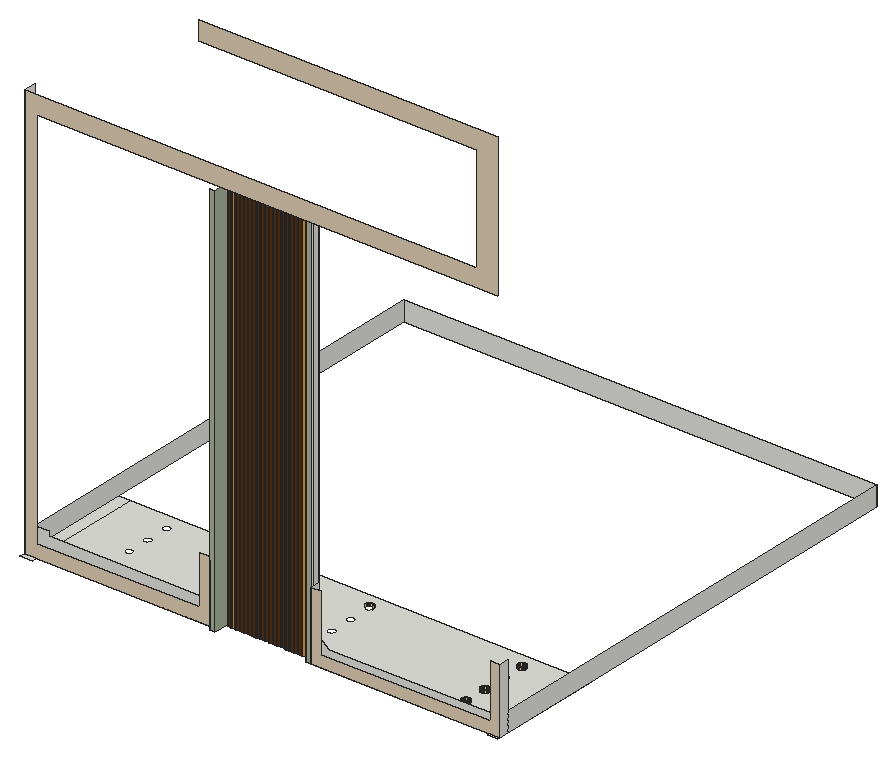
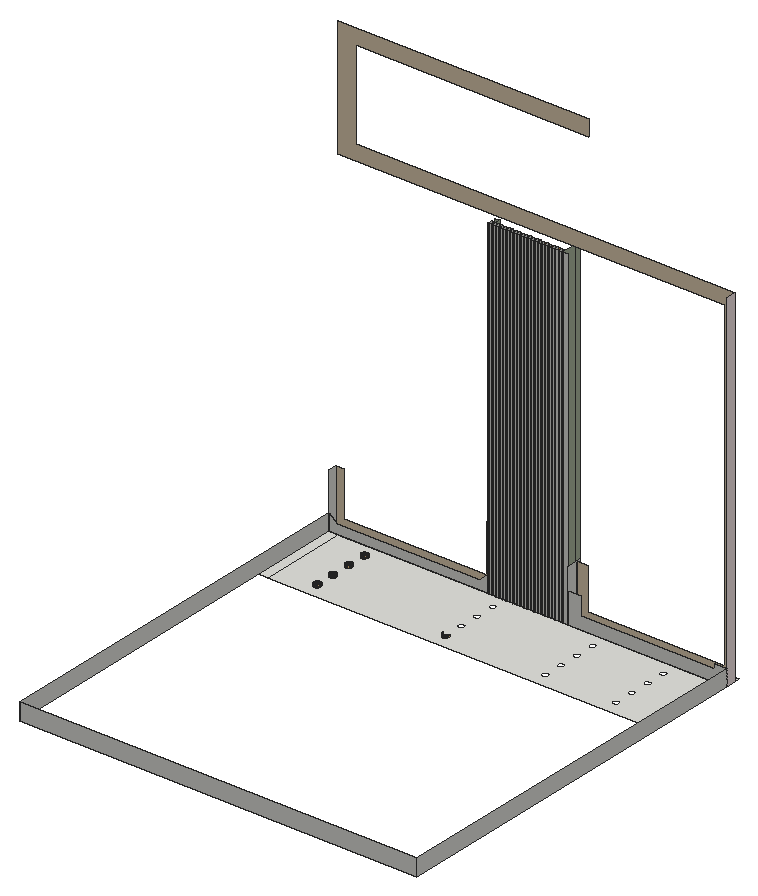
# SketchUp Ruby script. Lengths in inches.
U = 1.inch
M = Sketchup.active_model
def pt(a) = Geom::Point3d.new(a.map { |v| v * U })
def face(e, loops, mat)
  f = e.add_face(loops[0].map { |a| pt(a) })
  loops[1..].each { |l| e.add_face(l.map { |a| pt(a) }).erase! }
  f.material = f.back_material = mat if mat
  f
end
# faces: each face lists its corners as indices into pts; further lists are holes
def faces(e, pts, list, mat = nil) = list.each { |f| face(e, (f[0].is_a?(Array) ? f : [f]).map { |l| l.map { |i| pts[i] } }, mat) }
# xy, xz, yz: faces in a plane at the given z, y or x. An outline is a flat list of corners, or four numbers for a rectangle; further outlines are holes
def ring(l) = l.size == 4 ? [[l[0], l[1]], [l[2], l[1]], [l[2], l[3]], [l[0], l[3]]] : l.each_slice(2).to_a
def flat(e, list, mat, &to3) = list.each { |f| face(e, (f[0].is_a?(Array) ? f : [f]).map { |l| ring(l).map { |u, v| to3.(u, v) } }, mat) }
def xy(e, z, list, mat = nil) = flat(e, list, mat) { |x, y| [x, y, z] }
def xz(e, y, list, mat = nil) = flat(e, list, mat) { |x, z| [x, y, z] }
def yz(e, x, list, mat = nil) = flat(e, list, mat) { |y, z| [x, y, z] }
def lines(e, pts, list) = list.each { |a, b| e.add_line(pt(pts[a]), pt(pts[b])) }
# prism: a flat outline (further loops are holes) pulled along v
def prism(e, loops, v, mat = nil)
  f = face(e, loops, mat); d = Geom::Vector3d.new(v.map { |x| x * U })
  f.pushpull(f.normal.samedirection?(d) ? d.length : -d.length)
end
def box(e, o, s, mat = nil) = prism(e, [[o, [o[0] + s[0], o[1], o[2]], [o[0] + s[0], o[1] + s[1], o[2]], [o[0], o[1] + s[1], o[2]]]], [0, 0, s[2]], mat)
def at(x, y, z, deg = 0) = Geom::Transformation.translation(pt([x, y, z])) * Geom::Transformation.rotation(ORIGIN, Z_AXIS, deg.degrees)
def axes(o, x, y, z) = Geom::Transformation.new([*x, 0, *y, 0, *z, 0, *pt(o).to_a, 1])
def part(name) = M.definitions.add(name)
# library, detail: a bought-in or finely detailed component or shape, given as its bounding box
def library(name, o, s) = part(name).tap { |d| box(d.entities, o, s) }
def detail(e, o, s) = box(e.add_group.entities, o, s)
def put(e, d, t, mat = nil) = e.add_instance(d, t).tap { |i| i.material = mat if mat }
def group(e, t, mat = nil) = e.add_group.tap { |g| g.transformation = t; g.material = mat if mat }.entities
root = M.entities
M.materials.add("Generic").color = [90, 50, 18]
M.materials.add("Generic\#2").color = [245, 199, 133]
M.materials.add("Generic\#4").color = [232, 149, 60]
M.materials.add("Generic\#6").color = [223, 205, 179]
M.materials.add("Generic\#8").color = [168, 180, 155]
M.materials.add("Generic\#9").color = [246, 231, 231]
xy(root,120,[[2.3125,34.9375,15.4375,41],[204.09,35.5625,210.09,54.5625],[2.3125,41,15.4375,54.5625],[15.4375,41,204.09,54.5625],[497,41,507.875,43.625],
  [300.09,43.625,300.09,54.5625,300.47,54.5625,300.47,49.875,304.47,49.875,304.47,54.5625,306.09,54.5625,306.09,43.625],[306.09,43.625,497,54.5625],[497,43.625,507.875,54.5625],[211.72,49.875,215.72,54.5625],[300.47,49.875,304.47,54.5625],
  [2.3125,54.5625,15.4375,166.1875],[[15.4375,54.5625,497,166.1875],[448.19,68.72,449.28,68.86,450.29,69.28,451.15,69.95,451.82,70.8125,452.24,71.82,452.38,72.91,452.24,73.99,451.82,75,451.15,75.87,450.29,76.53,449.28,76.95,448.19,77.09,447.11,76.95,446.1,76.53,445.23,75.87,444.57,75,444.15,73.99,444,72.91,444.15,71.82,444.57,70.8125,445.23,69.95,446.1,69.28,447.11,68.86],[448.19,93.78,449.28,93.92,450.29,94.34,451.15,95.01,451.82,95.875,452.24,96.89,452.38,97.97,452.24,99.05,451.82,100.0625,451.15,100.93,450.29,101.6,449.28,102.01,448.19,102.16,447.11,102.01,446.1,101.6,445.23,100.93,444.57,100.0625,444.15,99.05,444,97.97,444.15,96.89,444.57,95.875,445.23,95.01,446.1,94.34,447.11,93.92],[68.07,93.78,69.15,93.92,70.16,94.34,71.03,95.01,71.69,95.875,72.11,96.89,72.25,97.97,72.11,99.05,71.69,100.0625,71.03,100.93,70.16,101.6,69.15,102.01,68.07,102.16,66.98,102.01,65.97,101.6,65.11,100.93,64.44,100.0625,64.02,99.05,63.88,97.97,64.02,96.89,64.44,95.875,65.11,95.01,65.97,94.34,66.98,93.92],[68.07,68.72,69.15,68.86,70.16,69.28,71.03,69.95,71.69,70.8125,72.11,71.82,72.25,72.91,72.11,73.99,71.69,75,71.03,75.87,70.16,76.53,69.15,76.95,68.07,77.09,66.98,76.95,65.97,76.53,65.11,75.87,64.44,75,64.02,73.99,63.88,72.91,64.02,71.82,64.44,70.8125,65.11,69.95,65.97,69.28,66.98,68.86],[157.88,93.78,158.96,93.92,159.97,94.34,160.84,95.01,161.51,95.875,161.92,96.89,162.07,97.97,161.92,99.05,161.51,100.0625,160.84,100.93,159.97,101.6,158.96,102.01,157.88,102.16,156.8,102.01,155.79,101.6,154.92,100.93,154.25,100.0625,153.83,99.05,153.69,97.97,153.83,96.89,154.25,95.875,154.92,95.01,155.79,94.34,156.8,93.92],[157.88,68.72,158.96,68.86,159.97,69.28,160.84,69.95,161.51,70.8125,161.92,71.82,162.07,72.91,161.92,73.99,161.51,75,160.84,75.87,159.97,76.53,158.96,76.95,157.88,77.09,156.8,76.95,155.79,76.53,154.92,75.87,154.25,75,153.83,73.99,153.69,72.91,153.83,71.82,154.25,70.8125,154.92,69.95,155.79,69.28,156.8,68.86],[284.88,93.78,285.96,93.92,286.97,94.34,287.84,95.01,288.51,95.875,288.92,96.89,289.07,97.97,288.92,99.05,288.51,100.0625,287.84,100.93,286.97,101.6,285.96,102.01,284.88,102.16,283.8,102.01,282.79,101.6,281.92,100.93,281.25,100.0625,280.83,99.05,280.69,97.97,280.83,96.89,281.25,95.875,281.92,95.01,282.79,94.34,283.8,93.92],[284.88,68.72,285.96,68.86,286.97,69.28,287.84,69.95,288.51,70.8125,288.92,71.82,289.07,72.91,288.92,73.99,288.51,75,287.84,75.87,286.97,76.53,285.96,76.95,284.88,77.09,283.8,76.95,282.79,76.53,281.92,75.87,281.25,75,280.83,73.99,280.69,72.91,280.83,71.82,281.25,70.8125,281.92,69.95,282.79,69.28,283.8,68.86],[448.19,118.84,449.28,118.99,450.29,119.41,451.15,120.07,451.82,120.9375,452.24,121.95,452.38,123.03,452.24,124.12,451.82,125.125,451.15,125.99,450.29,126.66,449.28,127.08,448.19,127.22,447.11,127.08,446.1,126.66,445.23,125.99,444.57,125.125,444.15,124.12,444,123.03,444.15,121.95,444.57,120.9375,445.23,120.07,446.1,119.41,447.11,118.99],[448.19,143.91,449.28,144.05,450.29,144.47,451.15,145.13,451.82,146,452.24,147.01,452.38,148.09,452.24,149.18,451.82,150.1875,451.15,151.06,450.29,151.72,449.28,152.14,448.19,152.28,447.11,152.14,446.1,151.72,445.23,151.06,444.57,150.1875,444.15,149.18,444,148.09,444.15,147.01,444.57,146,445.23,145.13,446.1,144.47,447.11,144.05],[68.07,143.91,69.15,144.05,70.16,144.47,71.03,145.13,71.69,146,72.11,147.01,72.25,148.09,72.11,149.18,71.69,150.1875,71.03,151.06,70.16,151.72,69.15,152.14,68.07,152.28,66.98,152.14,65.97,151.72,65.11,151.06,64.44,150.1875,64.02,149.18,63.88,148.09,64.02,147.01,64.44,146,65.11,145.13,65.97,144.47,66.98,144.05],[68.07,118.84,69.15,118.99,70.16,119.41,71.03,120.07,71.69,120.9375,72.11,121.95,72.25,123.03,72.11,124.12,71.69,125.125,71.03,125.99,70.16,126.66,69.15,127.08,68.07,127.22,66.98,127.08,65.97,126.66,65.11,125.99,64.44,125.125,64.02,124.12,63.88,123.03,64.02,121.95,64.44,120.9375,65.11,120.07,65.97,119.41,66.98,118.99],[157.88,143.91,158.96,144.05,159.97,144.47,160.84,145.13,161.51,146,161.92,147.01,162.07,148.09,161.92,149.18,161.51,150.1875,160.84,151.06,159.97,151.72,158.96,152.14,157.88,152.28,156.8,152.14,155.79,151.72,154.92,151.06,154.25,150.1875,153.83,149.18,153.69,148.09,153.83,147.01,154.25,146,154.92,145.13,155.79,144.47,156.8,144.05],[157.88,118.84,158.96,118.99,159.97,119.41,160.84,120.07,161.51,120.9375,161.92,121.95,162.07,123.03,161.92,124.12,161.51,125.125,160.84,125.99,159.97,126.66,158.96,127.08,157.88,127.22,156.8,127.08,155.79,126.66,154.92,125.99,154.25,125.125,153.83,124.12,153.69,123.03,153.83,121.95,154.25,120.9375,154.92,120.07,155.79,119.41,156.8,118.99],[284.88,143.91,285.96,144.05,286.97,144.47,287.84,145.13,288.51,146,288.92,147.01,289.07,148.09,288.92,149.18,288.51,150.1875,287.84,151.06,286.97,151.72,285.96,152.14,284.88,152.28,283.8,152.14,282.79,151.72,281.92,151.06,281.25,150.1875,280.83,149.18,280.69,148.09,280.83,147.01,281.25,146,281.92,145.13,282.79,144.47,283.8,144.05],[284.88,118.84,285.96,118.99,286.97,119.41,287.84,120.07,288.51,120.9375,288.92,121.95,289.07,123.03,288.92,124.12,288.51,125.125,287.84,125.99,286.97,126.66,285.96,127.08,284.88,127.22,283.8,127.08,282.79,126.66,281.92,125.99,281.25,125.125,280.83,124.12,280.69,123.03,280.83,121.95,281.25,120.9375,281.92,120.07,282.79,119.41,283.8,118.99]],[497,54.5625,507.875,166.1875]])
xz(root,35.5625,[[204.09,120,210.09,542.625]],"Generic\#8")
xz(root,41,[[2.3125,120,204.09,120,204.09,186.43,189,186.43,189,133.9375,15.3125,133.9375,15.3125,544.65,507.875,544.65,507.875,696.375,188.57,696.375,188.57,676.25,485.375,676.25,485.375,563.5,2.3125,563.5]],"Generic\#6")
xz(root,43.625,[[306.09,120,507.875,120,507.875,189.99,497.875,189.99,497.875,132.125,316.59,132.125,316.59,192.9375,306.09,192.9375]],"Generic\#6")
xz(root,43.625,[[300.09,120,306.09,542.625]],"Generic\#8")
xz(root,49.875,[[300.47,120,304.47,542.625]])
xz(root,49.875,[[296.03,119.25,300.03,542.625],[273.84,119.54,277.84,542.625],[278.28,119.54,282.28,542.625],[282.72,119.54,286.72,542.625],[287.16,119.54,291.16,542.625],
  [211.72,120,215.72,542.625],[220.59,120,224.59,542.625],[225.03,120,229.03,542.625],[229.47,120,233.47,542.625],[233.91,120,237.91,542.625],
  [238.34,120,242.34,542.625],[242.78,120,246.78,542.625],[247.22,120,251.22,542.625],[251.66,120,255.66,542.625],[256.09,120,260.09,542.625],
  [260.53,120,264.53,542.625],[264.97,120,268.97,542.625],[269.41,120,273.41,542.625]],"Generic")
xz(root,49.875,[[216.16,120,220.16,542.625]],"Generic\#4")
xz(root,54.5625,[[2.3125,120,2.3125,140.875,17.125,140.875,17.125,135.68,187.19,135.68,187.19,158.4375,204.09,158.4375,204.09,120],[204.09,120,210.09,542.625],[211.72,120,215.72,542.625],[215.72,120,216.16,542.625],[216.16,120,220.16,542.625],
  [220.16,120,220.59,542.625],[220.59,120,224.59,542.625],[224.59,120,225.03,542.625],[225.03,120,229.03,542.625],[229.03,120,229.47,542.625],
  [229.47,120,233.47,542.625],[233.47,120,233.91,542.625],[233.91,120,237.91,542.625],[237.91,120,238.34,542.625],[238.34,120,242.34,542.625],
  [242.34,120,242.78,542.625],[242.78,120,246.78,542.625],[246.78,120,247.22,542.625],[247.22,120,251.22,542.625],[251.22,120,251.66,542.625],
  [251.66,120,255.66,542.625],[255.66,120,256.09,542.625],[256.09,120,260.09,542.625],[260.09,120,260.53,542.625],[260.53,120,264.53,542.625],
  [264.53,120,264.97,542.625],[264.97,120,268.97,542.625],[268.97,120,269.41,542.625],[269.41,120,273.41,542.625],[273.41,120,273.84,542.625],
  [273.84,120,277.84,542.625],[277.84,120,278.28,542.625],[278.28,120,282.28,542.625],[282.28,120,282.72,542.625],[282.72,120,286.72,542.625],
  [286.72,120,287.16,542.625],[287.16,120,291.16,542.625],[291.16,120,291.59,542.625],[291.59,120,295.59,542.625],[295.59,120,296.03,542.625],
  [296.03,120,300.03,542.625],[300.03,120,300.09,542.625],[300.09,120,300.47,542.625],[300.47,120,304.47,542.625],[304.47,120,306.09,542.625],
  [306.09,120,306.09,140.875,316.59,132.125,497.875,132.125,507.875,140.875,507.875,120]])
xz(root,54.5625,[[210.09,120,211.72,542.625]],"Generic\#9")
xz(root,546.8125,[[2.3125,120,507.875,140.875]])
yz(root,2.3125,[[54.5625,120,546.8125,140.875]])
yz(root,2.3125,[[41,120,54.5625,563.5]],"Generic\#9")
yz(root,204.09,[[35.5625,120,41,186.43],[41,120,54.5625,186.43]])
yz(root,210.09,[[35.5625,120,54.5625,542.625]],"Generic\#8")
yz(root,211.72,[[49.875,120,54.5625,542.625]])
yz(root,215.72,[[49.875,120,54.5625,542.625]])
yz(root,216.16,[[49.875,120,54.5625,542.625]])
yz(root,220.16,[[49.875,120,54.5625,542.625]])
yz(root,220.59,[[49.875,120,54.5625,542.625]])
yz(root,224.59,[[49.875,120,54.5625,542.625]])
yz(root,225.03,[[49.875,120,54.5625,542.625]])
yz(root,229.03,[[49.875,120,54.5625,542.625]])
yz(root,229.47,[[49.875,120,54.5625,542.625]])
yz(root,233.47,[[49.875,120,54.5625,542.625]])
yz(root,233.91,[[49.875,120,54.5625,542.625]])
yz(root,237.91,[[49.875,120,54.5625,542.625]])
yz(root,238.34,[[49.875,120,54.5625,542.625]])
yz(root,242.34,[[49.875,120,54.5625,542.625]])
yz(root,242.78,[[49.875,120,54.5625,542.625]])
yz(root,246.78,[[49.875,120,54.5625,542.625]])
yz(root,247.22,[[49.875,120,54.5625,542.625]])
yz(root,251.22,[[49.875,120,54.5625,542.625]])
yz(root,251.66,[[49.875,120,54.5625,542.625]])
yz(root,255.66,[[49.875,120,54.5625,542.625]])
yz(root,256.09,[[49.875,120,54.5625,542.625]])
yz(root,260.09,[[49.875,120,54.5625,542.625]])
yz(root,260.53,[[49.875,120,54.5625,542.625]])
yz(root,264.53,[[49.875,120,54.5625,542.625]])
yz(root,264.97,[[49.875,120,54.5625,542.625]])
yz(root,268.97,[[49.875,120,54.5625,542.625]])
yz(root,269.41,[[49.875,120,54.5625,542.625]])
yz(root,273.41,[[49.875,120,54.5625,542.625]])
yz(root,273.84,[[49.875,119.54,54.5625,542.625]])
yz(root,277.84,[[49.875,119.54,54.5625,542.625]])
yz(root,278.28,[[49.875,119.54,54.5625,542.625]])
yz(root,282.28,[[49.875,119.54,54.5625,542.625]])
yz(root,282.72,[[49.875,119.54,54.5625,542.625]])
yz(root,286.72,[[49.875,119.54,54.5625,542.625]])
yz(root,287.16,[[49.875,119.54,54.5625,542.625]])
yz(root,291.16,[[49.875,119.54,54.5625,542.625]])
yz(root,291.59,[[50.11,119.54,49.875,542.625,54.5625,542.625,54.5625,120,54.8,119.54]])
yz(root,295.59,[[50.11,119.54,54.8,119.54,54.5625,120,54.5625,542.625,49.875,542.625]])
yz(root,296.03,[[49.875,119.25,54.5625,542.625]])
yz(root,300.03,[[49.875,119.25,54.5625,542.625]])
yz(root,300.09,[[43.625,120,54.5625,542.625]],"Generic\#8")
yz(root,300.47,[[49.875,120,54.5625,542.625]])
yz(root,304.47,[[49.875,120,54.5625,542.625]])
yz(root,306.09,[[43.625,120,54.5625,192.9375]])
yz(root,507.875,[[43.625,120,54.5625,189.99],[54.5625,120,546.8125,140.875]])
p = [[291.59,50.11,119.54],[295.59,50.11,119.54],[295.59,49.875,542.625],[291.59,49.875,542.625],[448.19,68.72,120],[447.11,68.86,120],
  [447.11,68.86,122.5625],[448.19,68.72,122.5625],[449.28,68.86,120],[449.28,68.86,122.5625],[446.1,69.28,120],[446.1,69.28,122.5625],
  [450.29,69.28,120],[450.29,69.28,122.5625],[445.23,69.95,120],[445.23,69.95,122.5625],[451.15,69.95,120],[451.15,69.95,122.5625],
  [444.57,70.8125,120],[444.57,70.8125,122.5625],[451.82,70.8125,120],[451.82,70.8125,122.5625],[444.15,71.82,120],[444.15,71.82,122.5625],
  [452.24,71.82,120],[452.24,71.82,122.5625],[444,72.91,120],[444,72.91,122.5625],[452.38,72.91,120],[452.38,72.91,122.5625],
  [444.15,73.99,120],[444.15,73.99,122.5625],[452.24,73.99,120],[452.24,73.99,122.5625],[444.57,75,120],[444.57,75,122.5625],
  [451.82,75,120],[451.82,75,122.5625],[445.23,75.87,120],[445.23,75.87,122.5625],[451.15,75.87,120],[451.15,75.87,122.5625],
  [446.1,76.53,120],[446.1,76.53,122.5625],[450.29,76.53,120],[450.29,76.53,122.5625],[447.11,76.95,120],[447.11,76.95,122.5625],
  [449.28,76.95,120],[449.28,76.95,122.5625],[448.19,77.09,120],[448.19,77.09,122.5625],[448.19,93.78,120],[447.11,93.92,120],
  [447.11,93.92,122.5625],[448.19,93.78,122.5625],[449.28,93.92,120],[449.28,93.92,122.5625],[446.1,94.34,120],[446.1,94.34,122.5625],
  [450.29,94.34,120],[450.29,94.34,122.5625],[445.23,95.01,120],[445.23,95.01,122.5625],[451.15,95.01,120],[451.15,95.01,122.5625],
  [444.57,95.875,120],[444.57,95.875,122.5625],[451.82,95.875,120],[451.82,95.875,122.5625],[444.15,96.89,120],[444.15,96.89,122.5625],
  [452.24,96.89,120],[452.24,96.89,122.5625],[444,97.97,120],[444,97.97,122.5625],[452.38,97.97,120],[452.38,97.97,122.5625],
  [444.15,99.05,120],[444.15,99.05,122.5625],[452.24,99.05,120],[452.24,99.05,122.5625],[444.57,100.0625,120],[444.57,100.0625,122.5625],
  [451.82,100.0625,120],[451.82,100.0625,122.5625],[445.23,100.93,120],[445.23,100.93,122.5625],[451.15,100.93,120],[451.15,100.93,122.5625],
  [446.1,101.6,120],[446.1,101.6,122.5625],[450.29,101.6,120],[450.29,101.6,122.5625],[447.11,102.01,120],[447.11,102.01,122.5625],
  [449.28,102.01,120],[449.28,102.01,122.5625],[448.19,102.16,120],[448.19,102.16,122.5625],[448.19,118.84,120],[447.11,118.99,120],
  [447.11,118.99,122.5625],[448.19,118.84,122.5625],[449.28,118.99,120],[449.28,118.99,122.5625],[446.1,119.41,120],[446.1,119.41,122.5625],
  [450.29,119.41,120],[450.29,119.41,122.5625],[445.23,120.07,120],[445.23,120.07,122.5625],[451.15,120.07,120],[451.15,120.07,122.5625],
  [444.57,120.9375,120],[444.57,120.9375,122.5625],[451.82,120.9375,120],[451.82,120.9375,122.5625],[444.15,121.95,120],[444.15,121.95,122.5625],
  [452.24,121.95,120],[452.24,121.95,122.5625],[444,123.03,120],[444,123.03,122.5625],[452.38,123.03,120],[452.38,123.03,122.5625],
  [444.15,124.12,120],[444.15,124.12,122.5625],[452.24,124.12,120],[452.24,124.12,122.5625],[444.57,125.125,120],[444.57,125.125,122.5625],
  [451.82,125.125,120],[451.82,125.125,122.5625],[445.23,125.99,120],[445.23,125.99,122.5625],[451.15,125.99,120],[451.15,125.99,122.5625],
  [446.1,126.66,120],[446.1,126.66,122.5625],[450.29,126.66,120],[450.29,126.66,122.5625],[447.11,127.08,120],[447.11,127.08,122.5625],
  [449.28,127.08,120],[449.28,127.08,122.5625],[448.19,127.22,120],[448.19,127.22,122.5625],[448.19,143.91,120],[447.11,144.05,120],
  [447.11,144.05,122.5625],[448.19,143.91,122.5625],[449.28,144.05,120],[449.28,144.05,122.5625],[446.1,144.47,120],[446.1,144.47,122.5625],
  [450.29,144.47,120],[450.29,144.47,122.5625],[445.23,145.13,120],[445.23,145.13,122.5625],[451.15,145.13,120],[451.15,145.13,122.5625],
  [444.57,146,120],[444.57,146,122.5625],[451.82,146,120],[451.82,146,122.5625],[444.15,147.01,120],[444.15,147.01,122.5625],
  [452.24,147.01,120],[452.24,147.01,122.5625],[280.83,147.01,120],[280.69,148.09,120],[280.69,148.09,122.5625],[280.83,147.01,122.5625],
  [444,148.09,120],[444,148.09,122.5625],[452.38,148.09,120],[452.38,148.09,122.5625],[280.83,149.18,120],[280.83,149.18,122.5625],
  [288.92,149.18,120],[289.07,148.09,120],[289.07,148.09,122.5625],[288.92,149.18,122.5625],[444.15,149.18,120],[444.15,149.18,122.5625],
  [452.24,149.18,120],[452.24,149.18,122.5625],[281.25,150.1875,120],[281.25,150.1875,122.5625],[288.51,150.1875,120],[288.51,150.1875,122.5625],
  [444.57,150.1875,120],[444.57,150.1875,122.5625],[451.82,150.1875,120],[451.82,150.1875,122.5625],[281.92,151.06,120],[281.92,151.06,122.5625],
  [287.84,151.06,120],[287.84,151.06,122.5625],[445.23,151.06,120],[445.23,151.06,122.5625],[451.15,151.06,120],[451.15,151.06,122.5625],
  [282.79,151.72,120],[282.79,151.72,122.5625],[286.97,151.72,120],[286.97,151.72,122.5625],[446.1,151.72,120],[446.1,151.72,122.5625],
  [450.29,151.72,120],[450.29,151.72,122.5625],[283.8,152.14,120],[283.8,152.14,122.5625],[285.96,152.14,120],[285.96,152.14,122.5625],
  [447.11,152.14,120],[447.11,152.14,122.5625],[449.28,152.14,120],[449.28,152.14,122.5625],[284.88,152.28,120],[284.88,152.28,122.5625],
  [448.19,152.28,120],[448.19,152.28,122.5625]]
faces(root,p,[[0,1,2,3]],"Generic\#4")
faces(root,p,[[4,5,6,7],[8,4,7,9],[5,10,11,6],[12,8,9,13],[10,14,15,11],[16,12,13,17],[14,18,19,15],[20,16,17,21],
  [18,22,23,19],[24,20,21,25],[22,26,27,23],[28,24,25,29],[26,30,31,27],[32,28,29,33],[30,34,35,31],[36,32,33,37],
  [34,38,39,35],[40,36,37,41],[38,42,43,39],[44,40,41,45],[42,46,47,43],[48,44,45,49],[46,50,51,47],[50,48,49,51],
  [52,53,54,55],[56,52,55,57],[53,58,59,54],[60,56,57,61],[58,62,63,59],[64,60,61,65],[62,66,67,63],[68,64,65,69],
  [66,70,71,67],[72,68,69,73],[70,74,75,71],[76,72,73,77],[74,78,79,75],[80,76,77,81],[78,82,83,79],[84,80,81,85],
  [82,86,87,83],[88,84,85,89],[86,90,91,87],[92,88,89,93],[90,94,95,91],[96,92,93,97],[94,98,99,95],[98,96,97,99],
  [100,101,102,103],[104,100,103,105],[101,106,107,102],[108,104,105,109],[106,110,111,107],[112,108,109,113],[110,114,115,111],[116,112,113,117],
  [114,118,119,115],[120,116,117,121],[118,122,123,119],[124,120,121,125],[122,126,127,123],[128,124,125,129],[126,130,131,127],[132,128,129,133],
  [130,134,135,131],[136,132,133,137],[134,138,139,135],[140,136,137,141],[138,142,143,139],[144,140,141,145],[142,146,147,143],[146,144,145,147],
  [148,149,150,151],[152,148,151,153],[149,154,155,150],[156,152,153,157],[154,158,159,155],[160,156,157,161],[158,162,163,159],[164,160,161,165],
  [162,166,167,163],[168,164,165,169],[170,171,172,173],[166,174,175,167],[176,168,169,177],[171,178,179,172],[180,181,182,183],[174,184,185,175],
  [186,176,177,187],[178,188,189,179],[190,180,183,191],[184,192,193,185],[194,186,187,195],[188,196,197,189],[198,190,191,199],[192,200,201,193],
  [202,194,195,203],[196,204,205,197],[206,198,199,207],[200,208,209,201],[210,202,203,211],[204,212,213,205],[214,206,207,215],[208,216,217,209],
  [218,210,211,219],[212,220,221,213],[220,214,215,221],[216,222,223,217],[222,218,219,223]],"Generic\#2")
